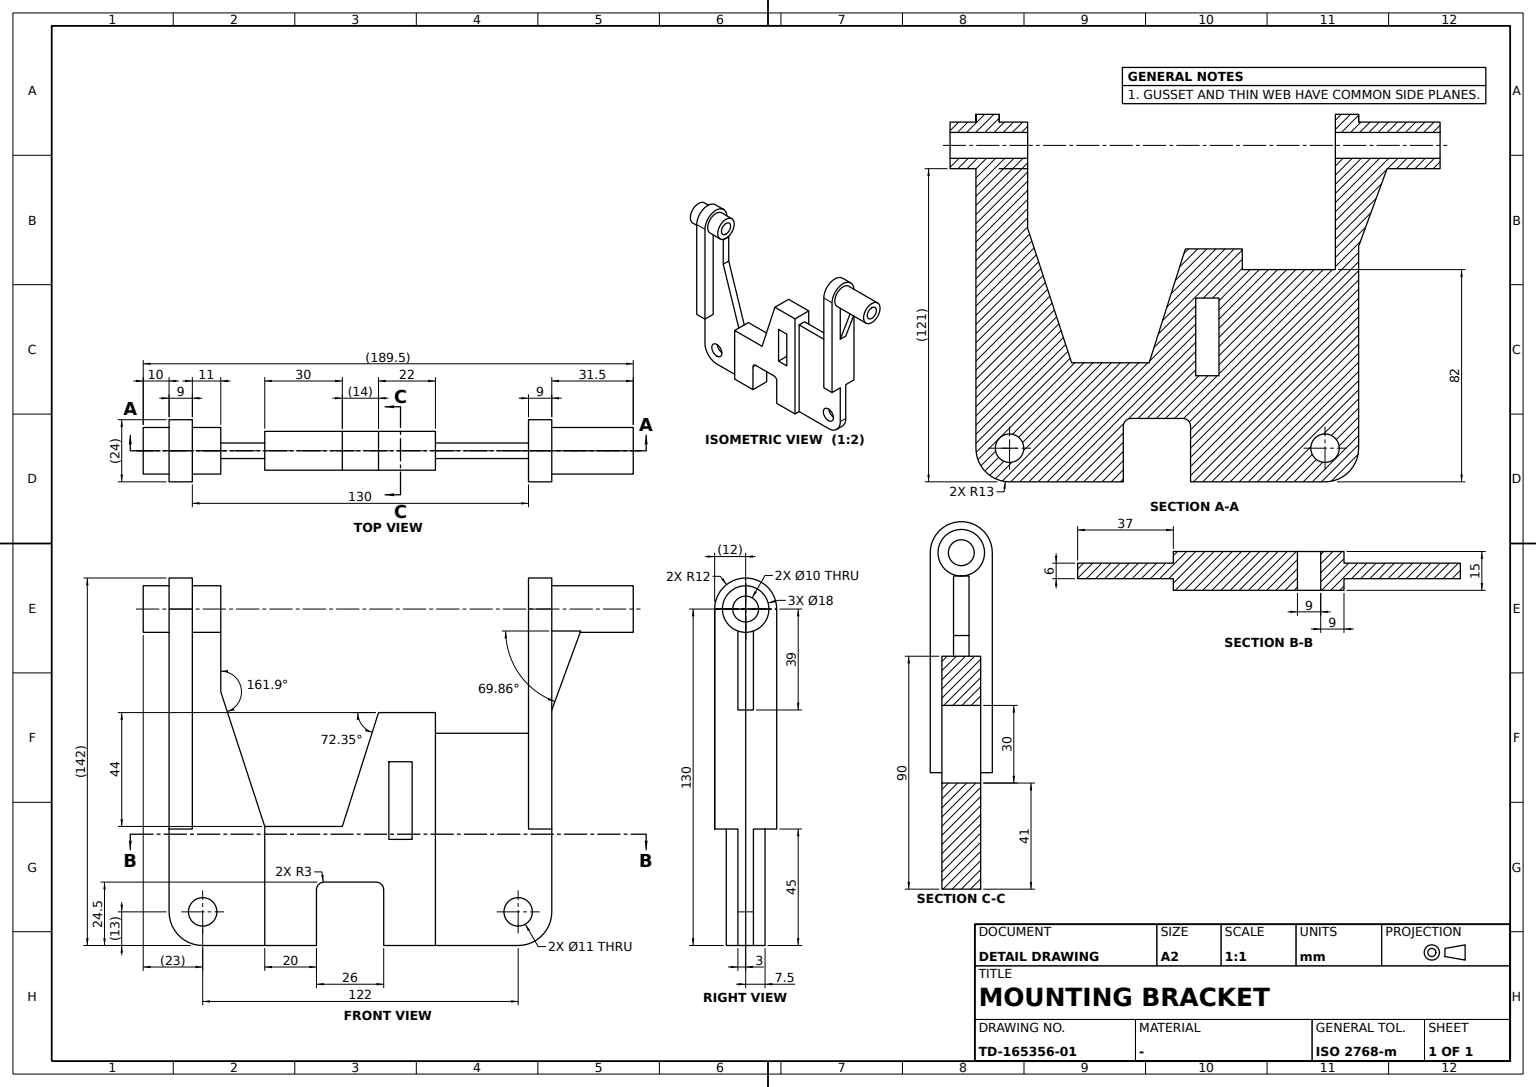
solid
v1 (-3,-50,98)
v2 (3,-50,98)
e1 v1 v2 LINE
v3 (-3,-50,121)
e2 v3 v1 LINE
v4 (3,-50,121)
e3 v3 v4 LINE
e4 v4 v2 LINE
face PLANE(AX(P(0,-50,121),D(0,-1,0),D(0,0,-1))) rev [-e1 -e2 e3 e4]
v5 (-7.5,24,71)
v6 (7.5,24,71)
e5 v5 v6 LINE
v7 (7.5,15,71)
e6 v7 v6 LINE
v8 (-7.5,15,71)
e7 v8 v7 LINE
e8 v8 v5 LINE
face PLANE(AX(P(0,15,71),D(0,0,-1),D(0,1,0))) [e5 -e6 -e7 e8]
v9 (-7.5,24,41)
v10 (7.5,24,41)
e9 v9 v10 LINE
v11 (-7.5,15,41)
e10 v9 v11 LINE
v12 (7.5,15,41)
e11 v11 v12 LINE
e12 v10 v12 LINE
face PLANE(AX(P(0,24,41),D(0,0,1),D(0,-1,0))) [-e9 e10 e11 -e12]
e13 v7 v12 LINE
e14 v8 v11 LINE
face PLANE(AX(P(0,15,71),D(0,-1,0),D(0,0,-1))) rev [e7 e13 -e11 -e14]
v13 (-3,-33,0)
v14 (-3,-57,0)
e15 v13 v14 LINE
v15 (-7.5,-33,0)
e16 v15 v13 LINE
v16 (-7.5,-13,0)
e17 v15 v16 LINE
v17 (7.5,-13,0)
e18 v16 v17 LINE
v18 (7.5,-33,0)
e19 v18 v17 LINE
v19 (3,-33,0)
e20 v19 v18 LINE
v20 (3,-57,0)
e21 v19 v20 LINE
e22 v14 v20 LINE
face PLANE(AX(P(0,-33,0),D(0,0,-1),D(0,1,0))) [-e15 -e16 e17 e18 -e19 -e20 e21 -e22]
v21 (-12,-61,45)
v22 (-12,-70,45)
e23 v21 v22 LINE
v23 (-3,-61,45)
e24 v21 v23 LINE
v24 (-3,-70,45)
e25 v24 v23 LINE
e26 v22 v24 LINE
face PLANE(AX(P(0,78,45),D(0,0,1),D(0,-1,0))) rev [-e23 e24 -e25 -e26]
v25 (-7.5,11,90)
v26 (-7.5,-3,46)
e27 v25 v26 LINE
v27 (-7.5,33,90)
e28 v27 v25 LINE
v28 (-7.5,33,0)
e29 v28 v27 LINE
v29 (-7.5,13,0)
e30 v29 v28 LINE
v30 (-7.5,13,21.5)
e31 v30 v29 LINE
v31 (-7.5,10,24.5)
e32 v30 v31 CIRCLE(AX(P(-7.5,10,21.5),D(1,0,0),D(0,0,-1)),3)
v32 (-7.5,-10,24.5)
e33 v32 v31 LINE
v33 (-7.5,-13,21.5)
e34 v32 v33 CIRCLE(AX(P(-7.5,-10,21.5),D(1,0,0),D(0,0,-1)),3)
e35 v16 v33 LINE
v34 (-7.5,-33,46)
e36 v34 v15 LINE
e37 v26 v34 LINE
e38 v9 v5 LINE
face PLANE(AX(P(-7.5,0,0),D(1,0,0),D(0,1,0))) rev [-e27 -e28 -e29 -e30 -e31 e32 -e33 e34 -e35 -e17 -e36 -e37] [-e8 e14 -e10 e38]
v35 (7.5,-13,21.5)
e39 v33 v35 LINE
e40 v17 v35 LINE
face PLANE(AX(P(0,-13,0),D(0,1,0),D(0,0,1))) [e39 -e40 -e18 e35]
v36 (7.5,13,21.5)
e41 v30 v36 LINE
v37 (7.5,13,0)
e42 v29 v37 LINE
e43 v36 v37 LINE
face PLANE(AX(P(0,13,21.5),D(0,-1,0),D(0,0,-1))) [-e41 e31 e42 -e43]
v38 (7.5,10,24.5)
e44 v31 v38 LINE
v39 (7.5,-10,24.5)
e45 v39 v38 LINE
e46 v32 v39 LINE
face PLANE(AX(P(0,-10,24.5),D(0,0,-1),D(0,1,0))) [e44 -e45 -e46 e33]
v40 (0,-80,125)
e47 v40 v40 CIRCLE(AX(P(0,-80,130),D(0,-1,0),D(0,0,-1)),5)
v41 (0,-50,125)
e48 v41 v41 CIRCLE(AX(P(0,-50,130),D(0,-1,0),D(0,0,-1)),5)
face CYL(AX(P(0,15.41,130),D(0,-1,0),D(1,0,0)),5) rev [e47] [-e48]
v42 (3,-33,46)
e49 v2 v42 LINE
v43 (3,-61,121)
e50 v43 v4 LINE
v44 (3,-61,45)
e51 v44 v43 LINE
v45 (3,-70,45)
e52 v45 v44 LINE
v46 (3,-70,13)
e53 v46 v45 LINE
e54 v46 v20 CIRCLE(AX(P(3,-57,13),D(1,0,0),D(0,0,-1)),13)
e55 v42 v19 LINE
v47 (3,-57,7.5)
e56 v47 v47 CIRCLE(AX(P(3,-57,13),D(1,0,0),D(0,0,-1)),5.5)
face PLANE(AX(P(3,0,0),D(1,0,0),D(0,1,0))) [-e49 -e4 -e50 -e51 -e52 -e53 e54 -e21 -e55] [-e56]
v48 (-12,69,45)
v49 (-12,69,130)
e57 v48 v49 LINE
v50 (-12,78,130)
e58 v49 v50 LINE
v51 (-12,78,45)
e59 v51 v50 LINE
e60 v48 v51 LINE
face PLANE(AX(P(-12,69,45),D(-1,0,0),D(0,0,1))) [e57 e58 -e59 -e60]
v52 (0,109.5,135)
e61 v52 v52 CIRCLE(AX(P(0,109.5,130),D(0,1,0),D(0,0,1)),5)
v53 (0,109.5,139)
e62 v53 v53 CIRCLE(AX(P(0,109.5,130),D(0,1,0),D(0,0,1)),9)
face PLANE(AX(P(0,109.5,0),D(0,1,0),D(-1,0,0))) [-e61] [e62]
v54 (3,78,13)
v55 (3,78,45)
e63 v54 v55 LINE
v56 (-3,78,13)
e64 v56 v54 LINE
v57 (-3,78,45)
e65 v56 v57 LINE
e66 v57 v51 LINE
v58 (12,78,130)
e67 v50 v58 CIRCLE(AX(P(0,78,130),D(0,1,0),D(0,0,1)),12)
v59 (12,78,45)
e68 v58 v59 LINE
e69 v59 v55 LINE
v60 (-3,78,121.514719)
v61 (3,78,121.514719)
e70 v60 v61 CIRCLE(AX(P(0,78,130),D(0,1,0),D(0,0,1)),9)
v62 (-3,78,91)
e71 v62 v60 LINE
v63 (3,78,91)
e72 v63 v62 LINE
e73 v63 v61 LINE
face PLANE(AX(P(0,78,13),D(0,1,0),D(0,0,1))) [-e63 -e64 e65 e66 e59 e67 e68 e69] [-e70 -e71 -e72 e73]
v64 (3,33,0)
v65 (3,33,82)
e74 v64 v65 LINE
v66 (3,65,0)
e75 v64 v66 LINE
e76 v66 v54 CIRCLE(AX(P(3,65,13),D(1,0,0),D(0,0,-1)),13)
v67 (3,69,45)
e77 v67 v55 LINE
v68 (3,69,82)
e78 v67 v68 LINE
e79 v68 v65 LINE
v69 (3,65,7.5)
e80 v69 v69 CIRCLE(AX(P(3,65,13),D(1,0,0),D(0,0,-1)),5.5)
face PLANE(AX(P(3,0,0),D(1,0,0),D(0,1,0))) [-e74 e75 e76 e63 -e77 e78 e79] [-e80]
v70 (-3,89.18873,121.514719)
e81 v62 v70 LINE
v71 (3,89.18873,121.514719)
e82 v70 v71 ELLIPSE(AX(P(0,92.3,130),D(0,0.938876316,-0.344254649),D(0,-0.344254649,-0.938876316)),9.585927,9) rev
e83 v71 v63 LINE
face PLANE(AX(P(0,89,121),D(0,0.938876316,-0.344254649),D(0,0.344254649,0.938876316))) [e81 e82 e83 e72]
v72 (-3,65,7.5)
e84 v72 v72 CIRCLE(AX(P(-3,65,13),D(1,0,0),D(0,0,-1)),5.5)
v73 (-3,65,0)
e85 v73 v56 CIRCLE(AX(P(-3,65,13),D(1,0,0),D(0,0,-1)),13)
v74 (-3,33,0)
e86 v74 v73 LINE
v75 (-3,33,82)
e87 v74 v75 LINE
v76 (-3,69,82)
e88 v76 v75 LINE
v77 (-3,69,45)
e89 v77 v76 LINE
e90 v77 v57 LINE
face PLANE(AX(P(-3,0,0),D(1,0,0),D(0,1,0))) rev [e84] [-e65 -e85 -e86 e87 -e88 -e89 e90]
e91 v36 v38 CIRCLE(AX(P(7.5,10,21.5),D(1,0,0),D(0,0,-1)),3)
face CYL(AX(P(0,10,21.5),D(1,0,0),D(0,1,0)),3) rev [-e32 e41 e91 -e44]
e92 v39 v35 CIRCLE(AX(P(7.5,-10,21.5),D(1,0,0),D(0,0,-1)),3)
face CYL(AX(P(0,-10,21.5),D(1,0,0),D(0,1,0)),3) rev [e92 -e39 -e34 e46]
v78 (12,69,45)
e93 v78 v59 LINE
e94 v78 v67 LINE
face PLANE(AX(P(0,78,45),D(0,0,1),D(0,-1,0))) rev [e77 -e69 -e93 e94]
e95 v73 v66 LINE
face CYL(AX(P(0,65,13),D(1,0,0),D(0,1,0)),13) [e85 e64 -e76 -e95]
e96 v77 v48 LINE
face PLANE(AX(P(0,78,45),D(0,0,1),D(0,-1,0))) rev [e96 e60 -e66 -e90]
v79 (0,-50,121)
e97 v79 v79 CIRCLE(AX(P(0,-50,130),D(0,-1,0),D(0,0,-1)),9) rev
v80 (0,-61,121)
e98 v80 v80 CIRCLE(AX(P(0,-61,130),D(0,1,0),D(0,0,1)),9)
face CYL(AX(P(0,-75,130),D(0,-1,0),D(1,0,0)),9) [-e97] [e98]
v81 (0,-70,139)
e99 v81 v81 CIRCLE(AX(P(0,-70,130),D(0,1,0),D(0,0,1)),9) rev
v82 (12,-70,45)
v83 (12,-70,130)
e100 v82 v83 LINE
v84 (-12,-70,130)
e101 v83 v84 CIRCLE(AX(P(0,-70,130),D(0,1,0),D(0,0,1)),12) rev
e102 v84 v22 LINE
v85 (-3,-70,13)
e103 v85 v24 LINE
e104 v85 v46 LINE
e105 v45 v82 LINE
face PLANE(AX(P(0,-70,13),D(0,1,0),D(0,0,1))) rev [-e99] [e100 e101 e102 e26 -e103 e104 e53 e105]
v86 (7.5,33,0)
e106 v64 v86 LINE
e107 v37 v86 LINE
e108 v28 v74 LINE
face PLANE(AX(P(0,-33,0),D(0,0,-1),D(0,1,0))) [-e75 e106 -e107 -e42 e30 e108 e86 e95]
v87 (-12,-61,130)
e109 v87 v84 LINE
e110 v87 v21 LINE
face PLANE(AX(P(-12,69,45),D(-1,0,0),D(0,0,1))) [e23 -e102 -e109 e110]
v88 (-3,-57,7.5)
e111 v88 v88 CIRCLE(AX(P(-3,-57,13),D(1,0,0),D(0,0,-1)),5.5)
face CYL(AX(P(0,-57,13),D(1,0,0),D(0,1,0)),5.5) rev [-e111] [e56]
v89 (12,-61,45)
e112 v89 v82 LINE
v90 (12,-61,130)
e113 v89 v90 LINE
e114 v90 v83 LINE
face PLANE(AX(P(12,69,130),D(1,0,0),D(0,0,-1))) [-e100 -e112 e113 e114]
v91 (0,-80,121)
e115 v91 v91 CIRCLE(AX(P(0,-80,130),D(0,-1,0),D(0,0,-1)),9)
face CYL(AX(P(0,-75,130),D(0,-1,0),D(1,0,0)),9) [e99] [-e115]
v92 (7.5,-33,46)
e116 v92 v18 LINE
e117 v42 v92 LINE
face PLANE(AX(P(0,-33,46),D(0,-1,0),D(0,0,-1))) [e55 e20 -e116 -e117]
e118 v61 v71 LINE
face PLANE(AX(P(3,0,0),D(1,0,0),D(0,1,0))) [-e118 -e73 -e83]
v93 (7.5,-3,46)
e119 v93 v92 LINE
e120 v26 v93 LINE
v94 (-3,-33,46)
e121 v34 v94 LINE
e122 v94 v42 LINE
face PLANE(AX(P(0,-3,46),D(0,0,1),D(0,-1,0))) [e117 -e119 -e120 e37 e121 e122]
e123 v1 v94 LINE
face PLANE(AX(P(0,-50,98),D(0,-0.950495325,-0.310738856),D(0,0.310738856,-0.950495325))) rev [-e123 e1 e49 -e122]
e124 v10 v6 LINE
face PLANE(AX(P(0,24,41),D(0,1,0),D(0,0,1))) rev [e124 -e5 -e38 e9]
face PLANE(AX(P(0,-80,0),D(0,-1,0),D(1,0,0))) [e115] [-e47]
e125 v90 v87 CIRCLE(AX(P(0,-61,130),D(0,1,0),D(0,0,1)),12) rev
face CYL(AX(P(0,73.5,130),D(0,1,0),D(-1,0,0)),12) [e109 -e101 -e114 e125]
e126 v85 v14 CIRCLE(AX(P(-3,-57,13),D(1,0,0),D(0,0,-1)),13)
v95 (-3,-61,121)
e127 v23 v95 LINE
e128 v95 v3 LINE
e129 v94 v13 LINE
face PLANE(AX(P(-3,0,0),D(1,0,0),D(0,1,0))) rev [e111] [-e126 e103 e25 e127 e128 e2 e123 e129 e15]
v96 (0,69,135)
e130 v96 v96 CIRCLE(AX(P(0,69,130),D(0,1,0),D(0,0,1)),5)
v97 (12,69,130)
e131 v97 v78 LINE
e132 v49 v97 CIRCLE(AX(P(0,69,130),D(0,1,0),D(0,0,1)),12)
e133 v76 v68 LINE
face PLANE(AX(P(0,69,45),D(0,1,0),D(0,0,1))) rev [e130] [-e131 -e132 -e57 -e96 e89 e133 -e78 -e94]
face PLANE(AX(P(0,-33,46),D(0,-1,0),D(0,0,-1))) [-e121 e36 e16 -e129]
e134 v75 v65 LINE
face PLANE(AX(P(0,69,82),D(0,0,1),D(0,-1,0))) [e134 -e79 -e133 e88]
e135 v97 v58 LINE
face CYL(AX(P(0,73.5,130),D(0,1,0),D(-1,0,0)),12) [e135 -e67 -e58 e132]
v98 (7.5,33,90)
e136 v27 v98 LINE
v99 (7.5,11,90)
e137 v25 v99 LINE
e138 v98 v99 LINE
face PLANE(AX(P(0,33,90),D(0,0,1),D(0,-1,0))) [-e136 e28 e137 -e138]
e139 v60 v70 LINE
face PLANE(AX(P(-3,0,0),D(1,0,0),D(0,1,0))) rev [-e81 e71 e139]
face CYL(AX(P(0,-75,130),D(0,-1,0),D(1,0,0)),9) [e70 e118 -e82 -e139] [-e62]
e140 v86 v98 LINE
face PLANE(AX(P(0,33,0),D(0,1,0),D(0,0,1))) [e136 -e140 -e106 e74 -e134 -e87 -e108 e29]
e141 v44 v89 LINE
face PLANE(AX(P(0,78,45),D(0,0,1),D(0,-1,0))) rev [e52 e141 e112 -e105]
e142 v80 v43 LINE
e143 v95 v80 LINE
face PLANE(AX(P(0,-61,121),D(0,0,-1),D(0,1,0))) rev [e142 e50 -e3 -e128 e143]
e144 v99 v93 LINE
face PLANE(AX(P(0,11,90),D(0,-0.95292578,0.303203657),D(0,-0.303203657,-0.95292578))) [e27 e120 -e144 -e137]
face CYL(AX(P(0,15.41,130),D(0,-1,0),D(1,0,0)),5) rev [e61] [-e130]
face PLANE(AX(P(0,-50,121),D(0,-1,0),D(0,0,-1))) rev [e48] [e97]
face CYL(AX(P(0,-57,13),D(1,0,0),D(0,1,0)),13) [-e54 -e104 e126 e22]
face CYL(AX(P(0,65,13),D(1,0,0),D(0,1,0)),5.5) rev [e80] [-e84]
face PLANE(AX(P(0,-61,45),D(0,1,0),D(0,0,1))) [-e125 -e113 -e141 e51 -e142 -e98 -e143 -e127 -e24 -e110]
face PLANE(AX(P(12,69,130),D(1,0,0),D(0,0,-1))) [e93 -e68 -e135 e131]
face PLANE(AX(P(7.5,0,0),D(1,0,0),D(0,1,0))) [-e124 e12 -e13 e6] [e40 -e92 e45 -e91 e43 e107 e140 e138 e144 e119 e116 e19]
